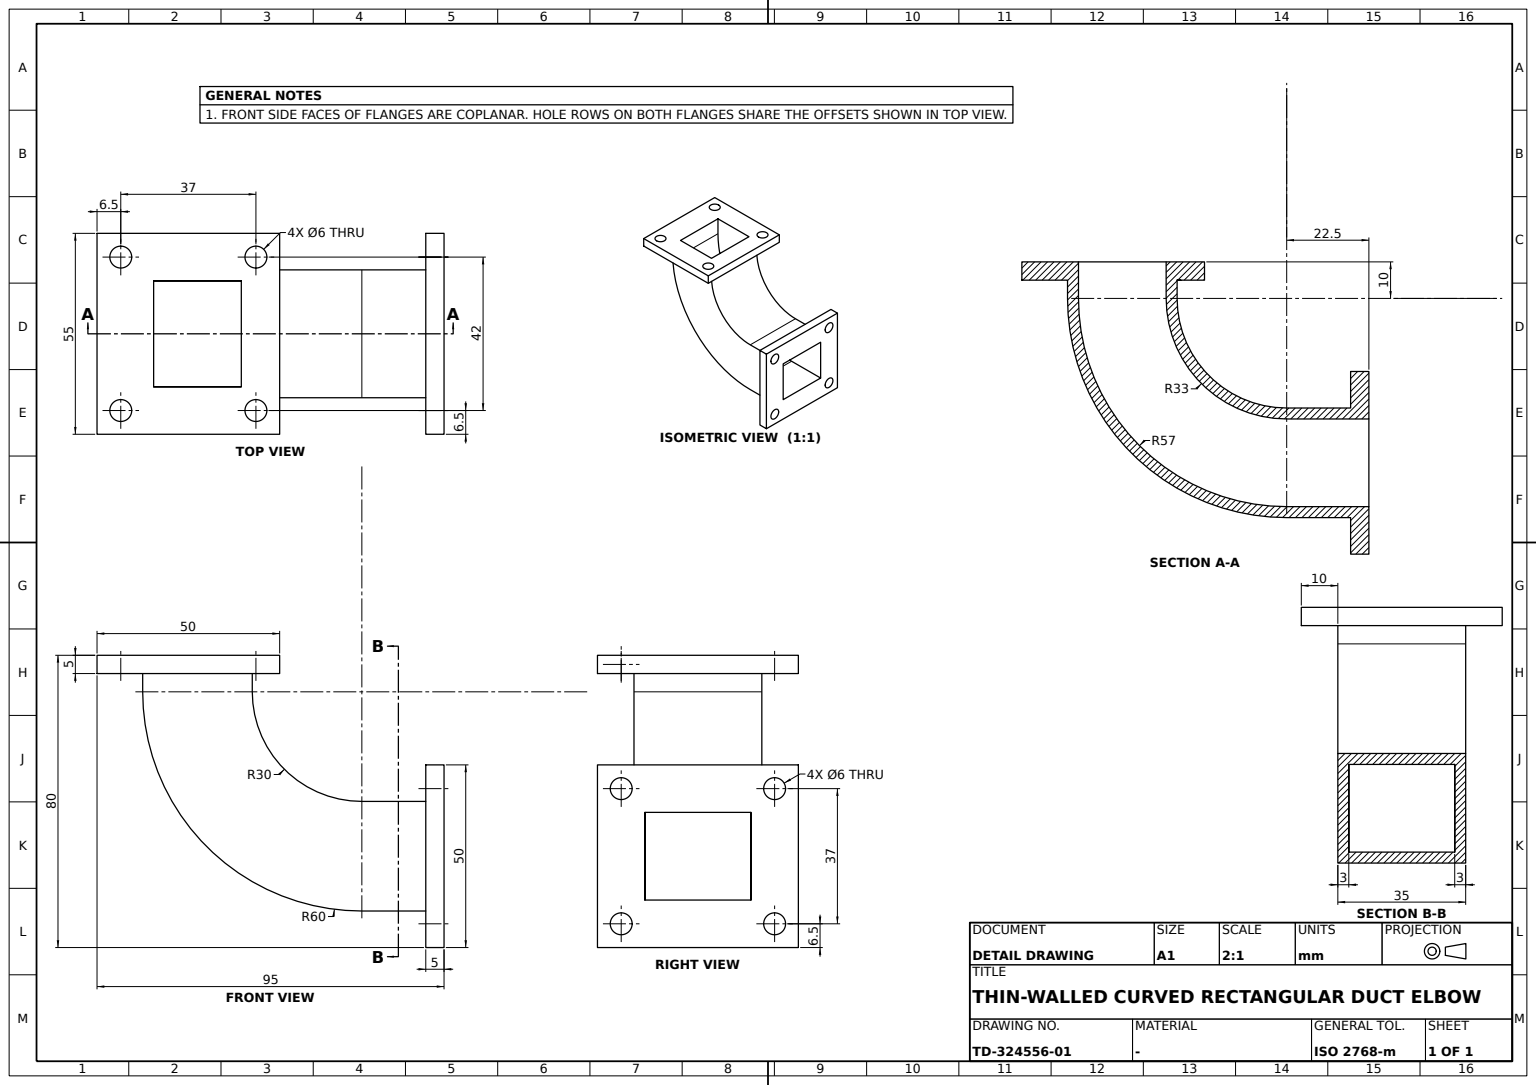
ISO-10303-21;
HEADER;
FILE_DESCRIPTION((''),'2;1');
FILE_NAME('','',(''),(''),'','','');
FILE_SCHEMA(('AUTOMOTIVE_DESIGN'));
ENDSEC;
DATA;
#1=APPLICATION_CONTEXT('');
#2=PRODUCT_CONTEXT('',#1,'mechanical');
#3=PRODUCT('','','',(#2));
#4=PRODUCT_DEFINITION_FORMATION('','',#3);
#5=PRODUCT_DEFINITION_CONTEXT('',#1,'design');
#6=PRODUCT_DEFINITION('','',#4,#5);
#7=PRODUCT_DEFINITION_SHAPE('','',#6);
#8=(LENGTH_UNIT()NAMED_UNIT(*)SI_UNIT(.MILLI.,.METRE.));
#9=(NAMED_UNIT(*)PLANE_ANGLE_UNIT()SI_UNIT($,.RADIAN.));
#10=(NAMED_UNIT(*)SI_UNIT($,.STERADIAN.)SOLID_ANGLE_UNIT());
#11=UNCERTAINTY_MEASURE_WITH_UNIT(LENGTH_MEASURE(1.E-05),#8,'distance_accuracy_value','');
#12=(GEOMETRIC_REPRESENTATION_CONTEXT(3)GLOBAL_UNCERTAINTY_ASSIGNED_CONTEXT((#11))GLOBAL_UNIT_ASSIGNED_CONTEXT((#8,#9,#10))REPRESENTATION_CONTEXT('',''));
#13=CARTESIAN_POINT('',(-24.,-18.5,0.));
#14=VERTEX_POINT('',#13);
#15=CARTESIAN_POINT('',(-18.,-18.5,0.));
#16=VERTEX_POINT('',#15);
#17=CARTESIAN_POINT('',(-21.,-18.5,0.));
#18=DIRECTION('',(0.,0.,-1.));
#19=DIRECTION('',(1.,0.,0.));
#20=AXIS2_PLACEMENT_3D('',#17,#18,#19);
#21=CIRCLE('',#20,3.);
#22=EDGE_CURVE('',#14,#16,#21,.T.);
#23=ORIENTED_EDGE('',*,*,#22,.F.);
#24=CARTESIAN_POINT('',(-24.,-18.5,-5.));
#25=VERTEX_POINT('',#24);
#26=CARTESIAN_POINT('',(-24.,-18.5,-2.5));
#27=DIRECTION('',(0.,0.,1.));
#28=VECTOR('',#27,1000.);
#29=LINE('',#26,#28);
#30=EDGE_CURVE('',#25,#14,#29,.T.);
#31=ORIENTED_EDGE('',*,*,#30,.F.);
#32=CARTESIAN_POINT('',(-18.,-18.5,-5.));
#33=VERTEX_POINT('',#32);
#34=CARTESIAN_POINT('',(-21.,-18.5,-5.));
#35=AXIS2_PLACEMENT_3D('',#34,#18,#19);
#36=CIRCLE('',#35,3.);
#37=EDGE_CURVE('',#25,#33,#36,.T.);
#38=ORIENTED_EDGE('',*,*,#37,.T.);
#39=CARTESIAN_POINT('',(-18.,-18.5,-2.5));
#40=LINE('',#39,#28);
#41=EDGE_CURVE('',#33,#16,#40,.T.);
#42=ORIENTED_EDGE('',*,*,#41,.T.);
#43=EDGE_LOOP('',(#23,#31,#38,#42));
#44=FACE_OUTER_BOUND('',#43,.T.);
#45=CARTESIAN_POINT('',(-21.,-18.5,-2.5));
#46=AXIS2_PLACEMENT_3D('',#45,#27,#19);
#47=CYLINDRICAL_SURFACE('',#46,3.);
#48=ADVANCED_FACE('',(#44),#47,.F.);
#49=CARTESIAN_POINT('',(-18.,-65.,31.5));
#50=VERTEX_POINT('',#49);
#51=CARTESIAN_POINT('',(-24.,-65.,31.5));
#52=VERTEX_POINT('',#51);
#53=CARTESIAN_POINT('',(-21.,-65.,31.5));
#54=DIRECTION('',(0.,-1.,0.));
#55=AXIS2_PLACEMENT_3D('',#53,#54,#19);
#56=CIRCLE('',#55,3.);
#57=EDGE_CURVE('',#50,#52,#56,.T.);
#58=ORIENTED_EDGE('',*,*,#57,.F.);
#59=CARTESIAN_POINT('',(-18.,-70.,31.5));
#60=VERTEX_POINT('',#59);
#61=CARTESIAN_POINT('',(-18.,-67.5,31.5));
#62=DIRECTION('',(0.,1.,0.));
#63=VECTOR('',#62,1000.);
#64=LINE('',#61,#63);
#65=EDGE_CURVE('',#60,#50,#64,.T.);
#66=ORIENTED_EDGE('',*,*,#65,.F.);
#67=CARTESIAN_POINT('',(-24.,-70.,31.5));
#68=VERTEX_POINT('',#67);
#69=CARTESIAN_POINT('',(-21.,-70.,31.5));
#70=AXIS2_PLACEMENT_3D('',#69,#54,#19);
#71=CIRCLE('',#70,3.);
#72=EDGE_CURVE('',#60,#68,#71,.T.);
#73=ORIENTED_EDGE('',*,*,#72,.T.);
#74=CARTESIAN_POINT('',(-24.,-67.5,31.5));
#75=LINE('',#74,#63);
#76=EDGE_CURVE('',#68,#52,#75,.T.);
#77=ORIENTED_EDGE('',*,*,#76,.T.);
#78=EDGE_LOOP('',(#58,#66,#73,#77));
#79=FACE_OUTER_BOUND('',#78,.T.);
#80=CARTESIAN_POINT('',(-21.,-67.5,31.5));
#81=AXIS2_PLACEMENT_3D('',#80,#62,#19);
#82=CYLINDRICAL_SURFACE('',#81,3.);
#83=ADVANCED_FACE('',(#79),#82,.F.);
#84=CARTESIAN_POINT('',(24.,-70.,68.5));
#85=VERTEX_POINT('',#84);
#86=CARTESIAN_POINT('',(24.,-65.,68.5));
#87=VERTEX_POINT('',#86);
#88=CARTESIAN_POINT('',(24.,-67.5,68.5));
#89=LINE('',#88,#63);
#90=EDGE_CURVE('',#85,#87,#89,.T.);
#91=ORIENTED_EDGE('',*,*,#90,.F.);
#92=CARTESIAN_POINT('',(18.,-70.,68.5));
#93=VERTEX_POINT('',#92);
#94=CARTESIAN_POINT('',(21.,-70.,68.5));
#95=AXIS2_PLACEMENT_3D('',#94,#54,#19);
#96=CIRCLE('',#95,3.);
#97=EDGE_CURVE('',#85,#93,#96,.T.);
#98=ORIENTED_EDGE('',*,*,#97,.T.);
#99=CARTESIAN_POINT('',(18.,-65.,68.5));
#100=VERTEX_POINT('',#99);
#101=CARTESIAN_POINT('',(18.,-67.5,68.5));
#102=LINE('',#101,#63);
#103=EDGE_CURVE('',#93,#100,#102,.T.);
#104=ORIENTED_EDGE('',*,*,#103,.T.);
#105=CARTESIAN_POINT('',(21.,-65.,68.5));
#106=AXIS2_PLACEMENT_3D('',#105,#54,#19);
#107=CIRCLE('',#106,3.);
#108=EDGE_CURVE('',#87,#100,#107,.T.);
#109=ORIENTED_EDGE('',*,*,#108,.F.);
#110=EDGE_LOOP('',(#91,#98,#104,#109));
#111=FACE_OUTER_BOUND('',#110,.T.);
#112=CARTESIAN_POINT('',(21.,-67.5,68.5));
#113=AXIS2_PLACEMENT_3D('',#112,#62,#19);
#114=CYLINDRICAL_SURFACE('',#113,3.);
#115=ADVANCED_FACE('',(#111),#114,.F.);
#116=ORIENTED_EDGE('',*,*,#108,.T.);
#117=EDGE_CURVE('',#100,#87,#107,.T.);
#118=ORIENTED_EDGE('',*,*,#117,.T.);
#119=EDGE_LOOP('',(#116,#118));
#120=FACE_BOUND('',#119,.T.);
#121=CARTESIAN_POINT('',(17.5,-65.,65.));
#122=VERTEX_POINT('',#121);
#123=CARTESIAN_POINT('',(-17.5,-65.,65.));
#124=VERTEX_POINT('',#123);
#125=CARTESIAN_POINT('',(0.,-65.,65.));
#126=DIRECTION('',(-1.,0.,0.));
#127=VECTOR('',#126,1000.);
#128=LINE('',#125,#127);
#129=EDGE_CURVE('',#122,#124,#128,.T.);
#130=ORIENTED_EDGE('',*,*,#129,.T.);
#131=CARTESIAN_POINT('',(-17.5,-65.,35.));
#132=VERTEX_POINT('',#131);
#133=CARTESIAN_POINT('',(-17.5,-65.,50.));
#134=VECTOR('',#18,1000.);
#135=LINE('',#133,#134);
#136=EDGE_CURVE('',#124,#132,#135,.T.);
#137=ORIENTED_EDGE('',*,*,#136,.T.);
#138=CARTESIAN_POINT('',(17.5,-65.,35.));
#139=VERTEX_POINT('',#138);
#140=CARTESIAN_POINT('',(0.,-65.,35.));
#141=VECTOR('',#19,1000.);
#142=LINE('',#140,#141);
#143=EDGE_CURVE('',#132,#139,#142,.T.);
#144=ORIENTED_EDGE('',*,*,#143,.T.);
#145=CARTESIAN_POINT('',(17.5,-65.,50.));
#146=LINE('',#145,#28);
#147=EDGE_CURVE('',#139,#122,#146,.T.);
#148=ORIENTED_EDGE('',*,*,#147,.T.);
#149=EDGE_LOOP('',(#130,#137,#144,#148));
#150=FACE_BOUND('',#149,.T.);
#151=CARTESIAN_POINT('',(-24.,-65.,68.5));
#152=VERTEX_POINT('',#151);
#153=CARTESIAN_POINT('',(-18.,-65.,68.5));
#154=VERTEX_POINT('',#153);
#155=CARTESIAN_POINT('',(-21.,-65.,68.5));
#156=AXIS2_PLACEMENT_3D('',#155,#54,#19);
#157=CIRCLE('',#156,3.);
#158=EDGE_CURVE('',#152,#154,#157,.T.);
#159=ORIENTED_EDGE('',*,*,#158,.T.);
#160=EDGE_CURVE('',#154,#152,#157,.T.);
#161=ORIENTED_EDGE('',*,*,#160,.T.);
#162=EDGE_LOOP('',(#159,#161));
#163=FACE_BOUND('',#162,.T.);
#164=CARTESIAN_POINT('',(-27.5,-65.,25.));
#165=VERTEX_POINT('',#164);
#166=CARTESIAN_POINT('',(27.5,-65.,25.));
#167=VERTEX_POINT('',#166);
#168=CARTESIAN_POINT('',(0.,-65.,25.));
#169=LINE('',#168,#141);
#170=EDGE_CURVE('',#165,#167,#169,.T.);
#171=ORIENTED_EDGE('',*,*,#170,.F.);
#172=CARTESIAN_POINT('',(-27.5,-65.,75.));
#173=VERTEX_POINT('',#172);
#174=CARTESIAN_POINT('',(-27.5,-65.,50.));
#175=LINE('',#174,#134);
#176=EDGE_CURVE('',#173,#165,#175,.T.);
#177=ORIENTED_EDGE('',*,*,#176,.F.);
#178=CARTESIAN_POINT('',(27.5,-65.,75.));
#179=VERTEX_POINT('',#178);
#180=CARTESIAN_POINT('',(0.,-65.,75.));
#181=LINE('',#180,#127);
#182=EDGE_CURVE('',#179,#173,#181,.T.);
#183=ORIENTED_EDGE('',*,*,#182,.F.);
#184=CARTESIAN_POINT('',(27.5,-65.,50.));
#185=LINE('',#184,#28);
#186=EDGE_CURVE('',#167,#179,#185,.T.);
#187=ORIENTED_EDGE('',*,*,#186,.F.);
#188=EDGE_LOOP('',(#171,#177,#183,#187));
#189=FACE_OUTER_BOUND('',#188,.T.);
#190=CARTESIAN_POINT('',(24.,-65.,31.5));
#191=VERTEX_POINT('',#190);
#192=CARTESIAN_POINT('',(18.,-65.,31.5));
#193=VERTEX_POINT('',#192);
#194=CARTESIAN_POINT('',(21.,-65.,31.5));
#195=AXIS2_PLACEMENT_3D('',#194,#54,#19);
#196=CIRCLE('',#195,3.);
#197=EDGE_CURVE('',#191,#193,#196,.T.);
#198=ORIENTED_EDGE('',*,*,#197,.T.);
#199=EDGE_CURVE('',#193,#191,#196,.T.);
#200=ORIENTED_EDGE('',*,*,#199,.T.);
#201=EDGE_LOOP('',(#198,#200));
#202=FACE_BOUND('',#201,.T.);
#203=EDGE_CURVE('',#52,#50,#56,.T.);
#204=ORIENTED_EDGE('',*,*,#203,.T.);
#205=ORIENTED_EDGE('',*,*,#57,.T.);
#206=EDGE_LOOP('',(#204,#205));
#207=FACE_BOUND('',#206,.T.);
#208=CARTESIAN_POINT('',(0.,-65.,0.));
#209=AXIS2_PLACEMENT_3D('',#208,#62,#126);
#210=PLANE('',#209);
#211=ADVANCED_FACE('',(#120,#150,#163,#189,#202,#207),#210,.T.);
#212=CARTESIAN_POINT('',(-27.5,25.,0.));
#213=VERTEX_POINT('',#212);
#214=CARTESIAN_POINT('',(-27.5,25.,-5.));
#215=VERTEX_POINT('',#214);
#216=CARTESIAN_POINT('',(-27.5,25.,-2.5));
#217=LINE('',#216,#134);
#218=EDGE_CURVE('',#213,#215,#217,.T.);
#219=ORIENTED_EDGE('',*,*,#218,.T.);
#220=CARTESIAN_POINT('',(-27.5,-25.,-5.));
#221=VERTEX_POINT('',#220);
#222=CARTESIAN_POINT('',(-27.5,0.,-5.));
#223=LINE('',#222,#63);
#224=EDGE_CURVE('',#221,#215,#223,.T.);
#225=ORIENTED_EDGE('',*,*,#224,.F.);
#226=CARTESIAN_POINT('',(-27.5,-25.,0.));
#227=VERTEX_POINT('',#226);
#228=CARTESIAN_POINT('',(-27.5,-25.,-2.5));
#229=LINE('',#228,#134);
#230=EDGE_CURVE('',#227,#221,#229,.T.);
#231=ORIENTED_EDGE('',*,*,#230,.F.);
#232=CARTESIAN_POINT('',(-27.5,0.,0.));
#233=LINE('',#232,#63);
#234=EDGE_CURVE('',#227,#213,#233,.T.);
#235=ORIENTED_EDGE('',*,*,#234,.T.);
#236=EDGE_LOOP('',(#219,#225,#231,#235));
#237=FACE_OUTER_BOUND('',#236,.T.);
#238=AXIS2_PLACEMENT_3D('',#164,#19,#27);
#239=PLANE('',#238);
#240=ADVANCED_FACE('',(#237),#239,.F.);
#241=CARTESIAN_POINT('',(-14.5,9.5,-5.));
#242=VERTEX_POINT('',#241);
#243=CARTESIAN_POINT('',(-14.5,9.5,5.));
#244=VERTEX_POINT('',#243);
#245=CARTESIAN_POINT('',(-14.5,9.5,0.));
#246=LINE('',#245,#28);
#247=EDGE_CURVE('',#242,#244,#246,.T.);
#248=ORIENTED_EDGE('',*,*,#247,.F.);
#249=CARTESIAN_POINT('',(14.5,9.5,-5.));
#250=VERTEX_POINT('',#249);
#251=CARTESIAN_POINT('',(0.,9.5,-5.));
#252=LINE('',#251,#141);
#253=EDGE_CURVE('',#242,#250,#252,.T.);
#254=ORIENTED_EDGE('',*,*,#253,.T.);
#255=CARTESIAN_POINT('',(14.5,9.5,5.));
#256=VERTEX_POINT('',#255);
#257=CARTESIAN_POINT('',(14.5,9.5,0.));
#258=LINE('',#257,#28);
#259=EDGE_CURVE('',#250,#256,#258,.T.);
#260=ORIENTED_EDGE('',*,*,#259,.T.);
#261=CARTESIAN_POINT('',(0.,9.5,5.));
#262=LINE('',#261,#127);
#263=EDGE_CURVE('',#256,#244,#262,.T.);
#264=ORIENTED_EDGE('',*,*,#263,.T.);
#265=EDGE_LOOP('',(#248,#254,#260,#264));
#266=FACE_OUTER_BOUND('',#265,.T.);
#267=AXIS2_PLACEMENT_3D('',#257,#62,#126);
#268=PLANE('',#267);
#269=ADVANCED_FACE('',(#266),#268,.F.);
#270=CARTESIAN_POINT('',(-14.5,-14.5,-5.));
#271=VERTEX_POINT('',#270);
#272=CARTESIAN_POINT('',(-14.5,-14.5,5.));
#273=VERTEX_POINT('',#272);
#274=CARTESIAN_POINT('',(-14.5,-14.5,0.));
#275=LINE('',#274,#28);
#276=EDGE_CURVE('',#271,#273,#275,.T.);
#277=ORIENTED_EDGE('',*,*,#276,.T.);
#278=CARTESIAN_POINT('',(14.5,-14.5,5.));
#279=VERTEX_POINT('',#278);
#280=CARTESIAN_POINT('',(0.,-14.5,5.));
#281=LINE('',#280,#141);
#282=EDGE_CURVE('',#273,#279,#281,.T.);
#283=ORIENTED_EDGE('',*,*,#282,.T.);
#284=CARTESIAN_POINT('',(14.5,-14.5,-5.));
#285=VERTEX_POINT('',#284);
#286=CARTESIAN_POINT('',(14.5,-14.5,0.));
#287=LINE('',#286,#28);
#288=EDGE_CURVE('',#285,#279,#287,.T.);
#289=ORIENTED_EDGE('',*,*,#288,.F.);
#290=CARTESIAN_POINT('',(0.,-14.5,-5.));
#291=LINE('',#290,#127);
#292=EDGE_CURVE('',#285,#271,#291,.T.);
#293=ORIENTED_EDGE('',*,*,#292,.T.);
#294=EDGE_LOOP('',(#277,#283,#289,#293));
#295=FACE_OUTER_BOUND('',#294,.T.);
#296=AXIS2_PLACEMENT_3D('',#274,#54,#19);
#297=PLANE('',#296);
#298=ADVANCED_FACE('',(#295),#297,.F.);
#299=CARTESIAN_POINT('',(-18.,-70.,68.5));
#300=VERTEX_POINT('',#299);
#301=CARTESIAN_POINT('',(-18.,-67.5,68.5));
#302=LINE('',#301,#63);
#303=EDGE_CURVE('',#300,#154,#302,.T.);
#304=ORIENTED_EDGE('',*,*,#303,.F.);
#305=CARTESIAN_POINT('',(-24.,-70.,68.5));
#306=VERTEX_POINT('',#305);
#307=CARTESIAN_POINT('',(-21.,-70.,68.5));
#308=AXIS2_PLACEMENT_3D('',#307,#54,#19);
#309=CIRCLE('',#308,3.);
#310=EDGE_CURVE('',#300,#306,#309,.T.);
#311=ORIENTED_EDGE('',*,*,#310,.T.);
#312=CARTESIAN_POINT('',(-24.,-67.5,68.5));
#313=LINE('',#312,#63);
#314=EDGE_CURVE('',#306,#152,#313,.T.);
#315=ORIENTED_EDGE('',*,*,#314,.T.);
#316=ORIENTED_EDGE('',*,*,#160,.F.);
#317=EDGE_LOOP('',(#304,#311,#315,#316));
#318=FACE_OUTER_BOUND('',#317,.T.);
#319=CARTESIAN_POINT('',(-21.,-67.5,68.5));
#320=AXIS2_PLACEMENT_3D('',#319,#62,#19);
#321=CYLINDRICAL_SURFACE('',#320,3.);
#322=ADVANCED_FACE('',(#318),#321,.F.);
#323=CARTESIAN_POINT('',(-14.5,-70.,38.));
#324=VERTEX_POINT('',#323);
#325=CARTESIAN_POINT('',(-14.5,-47.5,38.));
#326=VERTEX_POINT('',#325);
#327=CARTESIAN_POINT('',(-14.5,-58.75,38.));
#328=LINE('',#327,#63);
#329=EDGE_CURVE('',#324,#326,#328,.T.);
#330=ORIENTED_EDGE('',*,*,#329,.F.);
#331=CARTESIAN_POINT('',(14.5,-70.,38.));
#332=VERTEX_POINT('',#331);
#333=CARTESIAN_POINT('',(0.,-70.,38.));
#334=LINE('',#333,#141);
#335=EDGE_CURVE('',#324,#332,#334,.T.);
#336=ORIENTED_EDGE('',*,*,#335,.T.);
#337=CARTESIAN_POINT('',(14.5,-47.5,38.));
#338=VERTEX_POINT('',#337);
#339=CARTESIAN_POINT('',(14.5,-58.75,38.));
#340=LINE('',#339,#63);
#341=EDGE_CURVE('',#332,#338,#340,.T.);
#342=ORIENTED_EDGE('',*,*,#341,.T.);
#343=CARTESIAN_POINT('',(0.,-47.5,38.));
#344=LINE('',#343,#141);
#345=EDGE_CURVE('',#326,#338,#344,.T.);
#346=ORIENTED_EDGE('',*,*,#345,.F.);
#347=EDGE_LOOP('',(#330,#336,#342,#346));
#348=FACE_OUTER_BOUND('',#347,.T.);
#349=CARTESIAN_POINT('',(-14.5,-65.,38.));
#350=AXIS2_PLACEMENT_3D('',#349,#27,#19);
#351=PLANE('',#350);
#352=ADVANCED_FACE('',(#348),#351,.T.);
#353=ORIENTED_EDGE('',*,*,#263,.F.);
#354=CARTESIAN_POINT('',(14.5,-47.5,62.));
#355=VERTEX_POINT('',#354);
#356=CARTESIAN_POINT('',(14.5,-47.5,5.));
#357=AXIS2_PLACEMENT_3D('',#356,#19,#62);
#358=CIRCLE('',#357,57.);
#359=EDGE_CURVE('',#256,#355,#358,.T.);
#360=ORIENTED_EDGE('',*,*,#359,.T.);
#361=CARTESIAN_POINT('',(-14.5,-47.5,62.));
#362=VERTEX_POINT('',#361);
#363=CARTESIAN_POINT('',(0.,-47.5,62.));
#364=LINE('',#363,#127);
#365=EDGE_CURVE('',#355,#362,#364,.T.);
#366=ORIENTED_EDGE('',*,*,#365,.T.);
#367=CARTESIAN_POINT('',(-14.5,-47.5,5.));
#368=AXIS2_PLACEMENT_3D('',#367,#19,#62);
#369=CIRCLE('',#368,57.);
#370=EDGE_CURVE('',#244,#362,#369,.T.);
#371=ORIENTED_EDGE('',*,*,#370,.F.);
#372=EDGE_LOOP('',(#353,#360,#366,#371));
#373=FACE_OUTER_BOUND('',#372,.T.);
#374=CARTESIAN_POINT('',(0.,-47.5,5.));
#375=AXIS2_PLACEMENT_3D('',#374,#126,#62);
#376=CYLINDRICAL_SURFACE('',#375,57.);
#377=ADVANCED_FACE('',(#373),#376,.F.);
#378=CARTESIAN_POINT('',(-24.,18.5,-5.));
#379=VERTEX_POINT('',#378);
#380=CARTESIAN_POINT('',(-24.,18.5,0.));
#381=VERTEX_POINT('',#380);
#382=CARTESIAN_POINT('',(-24.,18.5,-2.5));
#383=LINE('',#382,#28);
#384=EDGE_CURVE('',#379,#381,#383,.T.);
#385=ORIENTED_EDGE('',*,*,#384,.F.);
#386=CARTESIAN_POINT('',(-18.,18.5,-5.));
#387=VERTEX_POINT('',#386);
#388=CARTESIAN_POINT('',(-21.,18.5,-5.));
#389=AXIS2_PLACEMENT_3D('',#388,#18,#19);
#390=CIRCLE('',#389,3.);
#391=EDGE_CURVE('',#379,#387,#390,.T.);
#392=ORIENTED_EDGE('',*,*,#391,.T.);
#393=CARTESIAN_POINT('',(-18.,18.5,0.));
#394=VERTEX_POINT('',#393);
#395=CARTESIAN_POINT('',(-18.,18.5,-2.5));
#396=LINE('',#395,#28);
#397=EDGE_CURVE('',#387,#394,#396,.T.);
#398=ORIENTED_EDGE('',*,*,#397,.T.);
#399=CARTESIAN_POINT('',(-21.,18.5,0.));
#400=AXIS2_PLACEMENT_3D('',#399,#18,#19);
#401=CIRCLE('',#400,3.);
#402=EDGE_CURVE('',#381,#394,#401,.T.);
#403=ORIENTED_EDGE('',*,*,#402,.F.);
#404=EDGE_LOOP('',(#385,#392,#398,#403));
#405=FACE_OUTER_BOUND('',#404,.T.);
#406=CARTESIAN_POINT('',(-21.,18.5,-2.5));
#407=AXIS2_PLACEMENT_3D('',#406,#27,#19);
#408=CYLINDRICAL_SURFACE('',#407,3.);
#409=ADVANCED_FACE('',(#405),#408,.F.);
#410=CARTESIAN_POINT('',(24.,-70.,31.5));
#411=VERTEX_POINT('',#410);
#412=CARTESIAN_POINT('',(18.,-70.,31.5));
#413=VERTEX_POINT('',#412);
#414=CARTESIAN_POINT('',(21.,-70.,31.5));
#415=AXIS2_PLACEMENT_3D('',#414,#54,#19);
#416=CIRCLE('',#415,3.);
#417=EDGE_CURVE('',#411,#413,#416,.T.);
#418=ORIENTED_EDGE('',*,*,#417,.T.);
#419=CARTESIAN_POINT('',(18.,-67.5,31.5));
#420=LINE('',#419,#63);
#421=EDGE_CURVE('',#413,#193,#420,.T.);
#422=ORIENTED_EDGE('',*,*,#421,.T.);
#423=ORIENTED_EDGE('',*,*,#197,.F.);
#424=CARTESIAN_POINT('',(24.,-67.5,31.5));
#425=LINE('',#424,#63);
#426=EDGE_CURVE('',#411,#191,#425,.T.);
#427=ORIENTED_EDGE('',*,*,#426,.F.);
#428=EDGE_LOOP('',(#418,#422,#423,#427));
#429=FACE_OUTER_BOUND('',#428,.T.);
#430=CARTESIAN_POINT('',(21.,-67.5,31.5));
#431=AXIS2_PLACEMENT_3D('',#430,#62,#19);
#432=CYLINDRICAL_SURFACE('',#431,3.);
#433=ADVANCED_FACE('',(#429),#432,.F.);
#434=CARTESIAN_POINT('',(14.5,-70.,62.));
#435=VERTEX_POINT('',#434);
#436=CARTESIAN_POINT('',(-14.5,-70.,62.));
#437=VERTEX_POINT('',#436);
#438=CARTESIAN_POINT('',(0.,-70.,62.));
#439=LINE('',#438,#127);
#440=EDGE_CURVE('',#435,#437,#439,.T.);
#441=ORIENTED_EDGE('',*,*,#440,.T.);
#442=CARTESIAN_POINT('',(-14.5,-58.75,62.));
#443=LINE('',#442,#63);
#444=EDGE_CURVE('',#437,#362,#443,.T.);
#445=ORIENTED_EDGE('',*,*,#444,.T.);
#446=ORIENTED_EDGE('',*,*,#365,.F.);
#447=CARTESIAN_POINT('',(14.5,-58.75,62.));
#448=LINE('',#447,#63);
#449=EDGE_CURVE('',#435,#355,#448,.T.);
#450=ORIENTED_EDGE('',*,*,#449,.F.);
#451=EDGE_LOOP('',(#441,#445,#446,#450));
#452=FACE_OUTER_BOUND('',#451,.T.);
#453=CARTESIAN_POINT('',(14.5,-65.,62.));
#454=AXIS2_PLACEMENT_3D('',#453,#18,#126);
#455=PLANE('',#454);
#456=ADVANCED_FACE('',(#452),#455,.T.);
#457=CARTESIAN_POINT('',(-17.5,-17.5,5.));
#458=VERTEX_POINT('',#457);
#459=CARTESIAN_POINT('',(-17.5,-47.5,35.));
#460=VERTEX_POINT('',#459);
#461=CARTESIAN_POINT('',(-17.5,-47.5,5.));
#462=AXIS2_PLACEMENT_3D('',#461,#19,#62);
#463=CIRCLE('',#462,30.);
#464=EDGE_CURVE('',#458,#460,#463,.T.);
#465=ORIENTED_EDGE('',*,*,#464,.T.);
#466=CARTESIAN_POINT('',(-17.5,-56.25,35.));
#467=LINE('',#466,#63);
#468=EDGE_CURVE('',#132,#460,#467,.T.);
#469=ORIENTED_EDGE('',*,*,#468,.F.);
#470=ORIENTED_EDGE('',*,*,#136,.F.);
#471=CARTESIAN_POINT('',(-17.5,-47.5,65.));
#472=VERTEX_POINT('',#471);
#473=CARTESIAN_POINT('',(-17.5,-56.25,65.));
#474=LINE('',#473,#63);
#475=EDGE_CURVE('',#124,#472,#474,.T.);
#476=ORIENTED_EDGE('',*,*,#475,.T.);
#477=CARTESIAN_POINT('',(-17.5,12.5,5.));
#478=VERTEX_POINT('',#477);
#479=CIRCLE('',#462,60.);
#480=EDGE_CURVE('',#478,#472,#479,.T.);
#481=ORIENTED_EDGE('',*,*,#480,.F.);
#482=CARTESIAN_POINT('',(-17.5,12.5,0.));
#483=VERTEX_POINT('',#482);
#484=CARTESIAN_POINT('',(-17.5,12.5,2.5));
#485=LINE('',#484,#28);
#486=EDGE_CURVE('',#483,#478,#485,.T.);
#487=ORIENTED_EDGE('',*,*,#486,.F.);
#488=CARTESIAN_POINT('',(-17.5,-17.5,0.));
#489=VERTEX_POINT('',#488);
#490=CARTESIAN_POINT('',(-17.5,-2.5,0.));
#491=VECTOR('',#54,1000.);
#492=LINE('',#490,#491);
#493=EDGE_CURVE('',#483,#489,#492,.T.);
#494=ORIENTED_EDGE('',*,*,#493,.T.);
#495=CARTESIAN_POINT('',(-17.5,-17.5,2.5));
#496=LINE('',#495,#28);
#497=EDGE_CURVE('',#489,#458,#496,.T.);
#498=ORIENTED_EDGE('',*,*,#497,.T.);
#499=EDGE_LOOP('',(#465,#469,#470,#476,#481,#487,#494,#498));
#500=FACE_OUTER_BOUND('',#499,.T.);
#501=AXIS2_PLACEMENT_3D('',#482,#126,#54);
#502=PLANE('',#501);
#503=ADVANCED_FACE('',(#500),#502,.T.);
#504=ORIENTED_EDGE('',*,*,#303,.T.);
#505=ORIENTED_EDGE('',*,*,#158,.F.);
#506=ORIENTED_EDGE('',*,*,#314,.F.);
#507=EDGE_CURVE('',#306,#300,#309,.T.);
#508=ORIENTED_EDGE('',*,*,#507,.T.);
#509=EDGE_LOOP('',(#504,#505,#506,#508));
#510=FACE_OUTER_BOUND('',#509,.T.);
#511=ADVANCED_FACE('',(#510),#321,.F.);
#512=CARTESIAN_POINT('',(27.5,25.,0.));
#513=VERTEX_POINT('',#512);
#514=CARTESIAN_POINT('',(27.5,-25.,0.));
#515=VERTEX_POINT('',#514);
#516=CARTESIAN_POINT('',(27.5,0.,0.));
#517=LINE('',#516,#491);
#518=EDGE_CURVE('',#513,#515,#517,.T.);
#519=ORIENTED_EDGE('',*,*,#518,.T.);
#520=CARTESIAN_POINT('',(27.5,-25.,-5.));
#521=VERTEX_POINT('',#520);
#522=CARTESIAN_POINT('',(27.5,-25.,-2.5));
#523=LINE('',#522,#134);
#524=EDGE_CURVE('',#515,#521,#523,.T.);
#525=ORIENTED_EDGE('',*,*,#524,.T.);
#526=CARTESIAN_POINT('',(27.5,25.,-5.));
#527=VERTEX_POINT('',#526);
#528=CARTESIAN_POINT('',(27.5,0.,-5.));
#529=LINE('',#528,#491);
#530=EDGE_CURVE('',#527,#521,#529,.T.);
#531=ORIENTED_EDGE('',*,*,#530,.F.);
#532=CARTESIAN_POINT('',(27.5,25.,-2.5));
#533=LINE('',#532,#134);
#534=EDGE_CURVE('',#513,#527,#533,.T.);
#535=ORIENTED_EDGE('',*,*,#534,.F.);
#536=EDGE_LOOP('',(#519,#525,#531,#535));
#537=FACE_OUTER_BOUND('',#536,.T.);
#538=AXIS2_PLACEMENT_3D('',#178,#126,#18);
#539=PLANE('',#538);
#540=ADVANCED_FACE('',(#537),#539,.F.);
#541=CARTESIAN_POINT('',(24.,-18.5,0.));
#542=VERTEX_POINT('',#541);
#543=CARTESIAN_POINT('',(18.,-18.5,0.));
#544=VERTEX_POINT('',#543);
#545=CARTESIAN_POINT('',(21.,-18.5,0.));
#546=AXIS2_PLACEMENT_3D('',#545,#18,#19);
#547=CIRCLE('',#546,3.);
#548=EDGE_CURVE('',#542,#544,#547,.T.);
#549=ORIENTED_EDGE('',*,*,#548,.T.);
#550=EDGE_CURVE('',#544,#542,#547,.T.);
#551=ORIENTED_EDGE('',*,*,#550,.T.);
#552=EDGE_LOOP('',(#549,#551));
#553=FACE_BOUND('',#552,.T.);
#554=EDGE_CURVE('',#394,#381,#401,.T.);
#555=ORIENTED_EDGE('',*,*,#554,.T.);
#556=ORIENTED_EDGE('',*,*,#402,.T.);
#557=EDGE_LOOP('',(#555,#556));
#558=FACE_BOUND('',#557,.T.);
#559=EDGE_CURVE('',#16,#14,#21,.T.);
#560=ORIENTED_EDGE('',*,*,#559,.T.);
#561=ORIENTED_EDGE('',*,*,#22,.T.);
#562=EDGE_LOOP('',(#560,#561));
#563=FACE_BOUND('',#562,.T.);
#564=CARTESIAN_POINT('',(17.5,12.5,0.));
#565=VERTEX_POINT('',#564);
#566=CARTESIAN_POINT('',(0.,12.5,0.));
#567=LINE('',#566,#127);
#568=EDGE_CURVE('',#565,#483,#567,.T.);
#569=ORIENTED_EDGE('',*,*,#568,.F.);
#570=CARTESIAN_POINT('',(17.5,-17.5,0.));
#571=VERTEX_POINT('',#570);
#572=CARTESIAN_POINT('',(17.5,-2.5,0.));
#573=LINE('',#572,#63);
#574=EDGE_CURVE('',#571,#565,#573,.T.);
#575=ORIENTED_EDGE('',*,*,#574,.F.);
#576=CARTESIAN_POINT('',(0.,-17.5,0.));
#577=LINE('',#576,#141);
#578=EDGE_CURVE('',#489,#571,#577,.T.);
#579=ORIENTED_EDGE('',*,*,#578,.F.);
#580=ORIENTED_EDGE('',*,*,#493,.F.);
#581=EDGE_LOOP('',(#569,#575,#579,#580));
#582=FACE_BOUND('',#581,.T.);
#583=CARTESIAN_POINT('',(0.,25.,0.));
#584=LINE('',#583,#141);
#585=EDGE_CURVE('',#213,#513,#584,.T.);
#586=ORIENTED_EDGE('',*,*,#585,.F.);
#587=ORIENTED_EDGE('',*,*,#234,.F.);
#588=CARTESIAN_POINT('',(0.,-25.,0.));
#589=LINE('',#588,#127);
#590=EDGE_CURVE('',#515,#227,#589,.T.);
#591=ORIENTED_EDGE('',*,*,#590,.F.);
#592=ORIENTED_EDGE('',*,*,#518,.F.);
#593=EDGE_LOOP('',(#586,#587,#591,#592));
#594=FACE_OUTER_BOUND('',#593,.T.);
#595=CARTESIAN_POINT('',(18.,18.5,0.));
#596=VERTEX_POINT('',#595);
#597=CARTESIAN_POINT('',(24.,18.5,0.));
#598=VERTEX_POINT('',#597);
#599=CARTESIAN_POINT('',(21.,18.5,0.));
#600=AXIS2_PLACEMENT_3D('',#599,#18,#19);
#601=CIRCLE('',#600,3.);
#602=EDGE_CURVE('',#596,#598,#601,.T.);
#603=ORIENTED_EDGE('',*,*,#602,.T.);
#604=EDGE_CURVE('',#598,#596,#601,.T.);
#605=ORIENTED_EDGE('',*,*,#604,.T.);
#606=EDGE_LOOP('',(#603,#605));
#607=FACE_BOUND('',#606,.T.);
#608=CARTESIAN_POINT('',(0.,-52.5,0.));
#609=AXIS2_PLACEMENT_3D('',#608,#18,#126);
#610=PLANE('',#609);
#611=ADVANCED_FACE('',(#553,#558,#563,#582,#594,#607),#610,.F.);
#612=ORIENTED_EDGE('',*,*,#449,.T.);
#613=ORIENTED_EDGE('',*,*,#359,.F.);
#614=ORIENTED_EDGE('',*,*,#259,.F.);
#615=CARTESIAN_POINT('',(14.5,-2.5,-5.));
#616=LINE('',#615,#491);
#617=EDGE_CURVE('',#250,#285,#616,.T.);
#618=ORIENTED_EDGE('',*,*,#617,.T.);
#619=ORIENTED_EDGE('',*,*,#288,.T.);
#620=CIRCLE('',#357,33.);
#621=EDGE_CURVE('',#279,#338,#620,.T.);
#622=ORIENTED_EDGE('',*,*,#621,.T.);
#623=ORIENTED_EDGE('',*,*,#341,.F.);
#624=CARTESIAN_POINT('',(14.5,-70.,50.));
#625=LINE('',#624,#28);
#626=EDGE_CURVE('',#332,#435,#625,.T.);
#627=ORIENTED_EDGE('',*,*,#626,.T.);
#628=EDGE_LOOP('',(#612,#613,#614,#618,#619,#622,#623,#627));
#629=FACE_OUTER_BOUND('',#628,.T.);
#630=AXIS2_PLACEMENT_3D('',#286,#19,#62);
#631=PLANE('',#630);
#632=ADVANCED_FACE('',(#629),#631,.F.);
#633=ORIENTED_EDGE('',*,*,#534,.T.);
#634=CARTESIAN_POINT('',(0.,25.,-5.));
#635=LINE('',#634,#141);
#636=EDGE_CURVE('',#215,#527,#635,.T.);
#637=ORIENTED_EDGE('',*,*,#636,.F.);
#638=ORIENTED_EDGE('',*,*,#218,.F.);
#639=ORIENTED_EDGE('',*,*,#585,.T.);
#640=EDGE_LOOP('',(#633,#637,#638,#639));
#641=FACE_OUTER_BOUND('',#640,.T.);
#642=AXIS2_PLACEMENT_3D('',#512,#54,#126);
#643=PLANE('',#642);
#644=ADVANCED_FACE('',(#641),#643,.F.);
#645=CARTESIAN_POINT('',(24.,-18.5,-5.));
#646=VERTEX_POINT('',#645);
#647=CARTESIAN_POINT('',(24.,-18.5,-2.5));
#648=LINE('',#647,#28);
#649=EDGE_CURVE('',#646,#542,#648,.T.);
#650=ORIENTED_EDGE('',*,*,#649,.T.);
#651=ORIENTED_EDGE('',*,*,#550,.F.);
#652=CARTESIAN_POINT('',(18.,-18.5,-5.));
#653=VERTEX_POINT('',#652);
#654=CARTESIAN_POINT('',(18.,-18.5,-2.5));
#655=LINE('',#654,#28);
#656=EDGE_CURVE('',#653,#544,#655,.T.);
#657=ORIENTED_EDGE('',*,*,#656,.F.);
#658=CARTESIAN_POINT('',(21.,-18.5,-5.));
#659=AXIS2_PLACEMENT_3D('',#658,#18,#19);
#660=CIRCLE('',#659,3.);
#661=EDGE_CURVE('',#653,#646,#660,.T.);
#662=ORIENTED_EDGE('',*,*,#661,.T.);
#663=EDGE_LOOP('',(#650,#651,#657,#662));
#664=FACE_OUTER_BOUND('',#663,.T.);
#665=CARTESIAN_POINT('',(21.,-18.5,-2.5));
#666=AXIS2_PLACEMENT_3D('',#665,#27,#19);
#667=CYLINDRICAL_SURFACE('',#666,3.);
#668=ADVANCED_FACE('',(#664),#667,.F.);
#669=ORIENTED_EDGE('',*,*,#444,.F.);
#670=CARTESIAN_POINT('',(-14.5,-70.,50.));
#671=LINE('',#670,#134);
#672=EDGE_CURVE('',#437,#324,#671,.T.);
#673=ORIENTED_EDGE('',*,*,#672,.T.);
#674=ORIENTED_EDGE('',*,*,#329,.T.);
#675=CIRCLE('',#368,33.);
#676=EDGE_CURVE('',#273,#326,#675,.T.);
#677=ORIENTED_EDGE('',*,*,#676,.F.);
#678=ORIENTED_EDGE('',*,*,#276,.F.);
#679=CARTESIAN_POINT('',(-14.5,-2.5,-5.));
#680=LINE('',#679,#63);
#681=EDGE_CURVE('',#271,#242,#680,.T.);
#682=ORIENTED_EDGE('',*,*,#681,.T.);
#683=ORIENTED_EDGE('',*,*,#247,.T.);
#684=ORIENTED_EDGE('',*,*,#370,.T.);
#685=EDGE_LOOP('',(#669,#673,#674,#677,#678,#682,#683,#684));
#686=FACE_OUTER_BOUND('',#685,.T.);
#687=AXIS2_PLACEMENT_3D('',#245,#126,#54);
#688=PLANE('',#687);
#689=ADVANCED_FACE('',(#686),#688,.F.);
#690=ORIENTED_EDGE('',*,*,#203,.F.);
#691=ORIENTED_EDGE('',*,*,#76,.F.);
#692=EDGE_CURVE('',#68,#60,#71,.T.);
#693=ORIENTED_EDGE('',*,*,#692,.T.);
#694=ORIENTED_EDGE('',*,*,#65,.T.);
#695=EDGE_LOOP('',(#690,#691,#693,#694));
#696=FACE_OUTER_BOUND('',#695,.T.);
#697=ADVANCED_FACE('',(#696),#82,.F.);
#698=ORIENTED_EDGE('',*,*,#554,.F.);
#699=ORIENTED_EDGE('',*,*,#397,.F.);
#700=EDGE_CURVE('',#387,#379,#390,.T.);
#701=ORIENTED_EDGE('',*,*,#700,.T.);
#702=ORIENTED_EDGE('',*,*,#384,.T.);
#703=EDGE_LOOP('',(#698,#699,#701,#702));
#704=FACE_OUTER_BOUND('',#703,.T.);
#705=ADVANCED_FACE('',(#704),#408,.F.);
#706=ORIENTED_EDGE('',*,*,#661,.F.);
#707=EDGE_CURVE('',#646,#653,#660,.T.);
#708=ORIENTED_EDGE('',*,*,#707,.F.);
#709=EDGE_LOOP('',(#706,#708));
#710=FACE_BOUND('',#709,.T.);
#711=ORIENTED_EDGE('',*,*,#700,.F.);
#712=ORIENTED_EDGE('',*,*,#391,.F.);
#713=EDGE_LOOP('',(#711,#712));
#714=FACE_BOUND('',#713,.T.);
#715=ORIENTED_EDGE('',*,*,#292,.F.);
#716=ORIENTED_EDGE('',*,*,#617,.F.);
#717=ORIENTED_EDGE('',*,*,#253,.F.);
#718=ORIENTED_EDGE('',*,*,#681,.F.);
#719=EDGE_LOOP('',(#715,#716,#717,#718));
#720=FACE_BOUND('',#719,.T.);
#721=ORIENTED_EDGE('',*,*,#530,.T.);
#722=CARTESIAN_POINT('',(0.,-25.,-5.));
#723=LINE('',#722,#127);
#724=EDGE_CURVE('',#521,#221,#723,.T.);
#725=ORIENTED_EDGE('',*,*,#724,.T.);
#726=ORIENTED_EDGE('',*,*,#224,.T.);
#727=ORIENTED_EDGE('',*,*,#636,.T.);
#728=EDGE_LOOP('',(#721,#725,#726,#727));
#729=FACE_OUTER_BOUND('',#728,.T.);
#730=CARTESIAN_POINT('',(24.,18.5,-5.));
#731=VERTEX_POINT('',#730);
#732=CARTESIAN_POINT('',(18.,18.5,-5.));
#733=VERTEX_POINT('',#732);
#734=CARTESIAN_POINT('',(21.,18.5,-5.));
#735=AXIS2_PLACEMENT_3D('',#734,#18,#19);
#736=CIRCLE('',#735,3.);
#737=EDGE_CURVE('',#731,#733,#736,.T.);
#738=ORIENTED_EDGE('',*,*,#737,.F.);
#739=EDGE_CURVE('',#733,#731,#736,.T.);
#740=ORIENTED_EDGE('',*,*,#739,.F.);
#741=EDGE_LOOP('',(#738,#740));
#742=FACE_BOUND('',#741,.T.);
#743=EDGE_CURVE('',#33,#25,#36,.T.);
#744=ORIENTED_EDGE('',*,*,#743,.F.);
#745=ORIENTED_EDGE('',*,*,#37,.F.);
#746=EDGE_LOOP('',(#744,#745));
#747=FACE_BOUND('',#746,.T.);
#748=CARTESIAN_POINT('',(0.,0.,-5.));
#749=AXIS2_PLACEMENT_3D('',#748,#18,#19);
#750=PLANE('',#749);
#751=ADVANCED_FACE('',(#710,#714,#720,#729,#742,#747),#750,.T.);
#752=CARTESIAN_POINT('',(27.5,-70.,25.));
#753=VERTEX_POINT('',#752);
#754=CARTESIAN_POINT('',(27.5,-70.,75.));
#755=VERTEX_POINT('',#754);
#756=CARTESIAN_POINT('',(27.5,-70.,50.));
#757=LINE('',#756,#28);
#758=EDGE_CURVE('',#753,#755,#757,.T.);
#759=ORIENTED_EDGE('',*,*,#758,.F.);
#760=CARTESIAN_POINT('',(27.5,-67.5,25.));
#761=LINE('',#760,#491);
#762=EDGE_CURVE('',#167,#753,#761,.T.);
#763=ORIENTED_EDGE('',*,*,#762,.F.);
#764=ORIENTED_EDGE('',*,*,#186,.T.);
#765=CARTESIAN_POINT('',(27.5,-67.5,75.));
#766=LINE('',#765,#491);
#767=EDGE_CURVE('',#179,#755,#766,.T.);
#768=ORIENTED_EDGE('',*,*,#767,.T.);
#769=EDGE_LOOP('',(#759,#763,#764,#768));
#770=FACE_OUTER_BOUND('',#769,.T.);
#771=ADVANCED_FACE('',(#770),#539,.F.);
#772=CARTESIAN_POINT('',(17.5,-47.5,35.));
#773=VERTEX_POINT('',#772);
#774=CARTESIAN_POINT('',(17.5,-56.25,35.));
#775=LINE('',#774,#63);
#776=EDGE_CURVE('',#139,#773,#775,.T.);
#777=ORIENTED_EDGE('',*,*,#776,.F.);
#778=ORIENTED_EDGE('',*,*,#143,.F.);
#779=ORIENTED_EDGE('',*,*,#468,.T.);
#780=CARTESIAN_POINT('',(0.,-47.5,35.));
#781=LINE('',#780,#141);
#782=EDGE_CURVE('',#460,#773,#781,.T.);
#783=ORIENTED_EDGE('',*,*,#782,.T.);
#784=EDGE_LOOP('',(#777,#778,#779,#783));
#785=FACE_OUTER_BOUND('',#784,.T.);
#786=AXIS2_PLACEMENT_3D('',#131,#27,#19);
#787=PLANE('',#786);
#788=ADVANCED_FACE('',(#785),#787,.F.);
#789=ORIENTED_EDGE('',*,*,#230,.T.);
#790=ORIENTED_EDGE('',*,*,#724,.F.);
#791=ORIENTED_EDGE('',*,*,#524,.F.);
#792=ORIENTED_EDGE('',*,*,#590,.T.);
#793=EDGE_LOOP('',(#789,#790,#791,#792));
#794=FACE_OUTER_BOUND('',#793,.T.);
#795=AXIS2_PLACEMENT_3D('',#226,#62,#19);
#796=PLANE('',#795);
#797=ADVANCED_FACE('',(#794),#796,.F.);
#798=ORIENTED_EDGE('',*,*,#602,.F.);
#799=CARTESIAN_POINT('',(18.,18.5,-2.5));
#800=LINE('',#799,#28);
#801=EDGE_CURVE('',#733,#596,#800,.T.);
#802=ORIENTED_EDGE('',*,*,#801,.F.);
#803=ORIENTED_EDGE('',*,*,#739,.T.);
#804=CARTESIAN_POINT('',(24.,18.5,-2.5));
#805=LINE('',#804,#28);
#806=EDGE_CURVE('',#731,#598,#805,.T.);
#807=ORIENTED_EDGE('',*,*,#806,.T.);
#808=EDGE_LOOP('',(#798,#802,#803,#807));
#809=FACE_OUTER_BOUND('',#808,.T.);
#810=CARTESIAN_POINT('',(21.,18.5,-2.5));
#811=AXIS2_PLACEMENT_3D('',#810,#27,#19);
#812=CYLINDRICAL_SURFACE('',#811,3.);
#813=ADVANCED_FACE('',(#809),#812,.F.);
#814=ORIENTED_EDGE('',*,*,#41,.F.);
#815=ORIENTED_EDGE('',*,*,#743,.T.);
#816=ORIENTED_EDGE('',*,*,#30,.T.);
#817=ORIENTED_EDGE('',*,*,#559,.F.);
#818=EDGE_LOOP('',(#814,#815,#816,#817));
#819=FACE_OUTER_BOUND('',#818,.T.);
#820=ADVANCED_FACE('',(#819),#47,.F.);
#821=ORIENTED_EDGE('',*,*,#170,.T.);
#822=ORIENTED_EDGE('',*,*,#762,.T.);
#823=CARTESIAN_POINT('',(-27.5,-70.,25.));
#824=VERTEX_POINT('',#823);
#825=CARTESIAN_POINT('',(0.,-70.,25.));
#826=LINE('',#825,#141);
#827=EDGE_CURVE('',#824,#753,#826,.T.);
#828=ORIENTED_EDGE('',*,*,#827,.F.);
#829=CARTESIAN_POINT('',(-27.5,-67.5,25.));
#830=LINE('',#829,#491);
#831=EDGE_CURVE('',#165,#824,#830,.T.);
#832=ORIENTED_EDGE('',*,*,#831,.F.);
#833=EDGE_LOOP('',(#821,#822,#828,#832));
#834=FACE_OUTER_BOUND('',#833,.T.);
#835=AXIS2_PLACEMENT_3D('',#166,#27,#126);
#836=PLANE('',#835);
#837=ADVANCED_FACE('',(#834),#836,.F.);
#838=CARTESIAN_POINT('',(17.5,-47.5,65.));
#839=VERTEX_POINT('',#838);
#840=CARTESIAN_POINT('',(0.,-47.5,65.));
#841=LINE('',#840,#127);
#842=EDGE_CURVE('',#839,#472,#841,.T.);
#843=ORIENTED_EDGE('',*,*,#842,.F.);
#844=CARTESIAN_POINT('',(17.5,12.5,5.));
#845=VERTEX_POINT('',#844);
#846=CARTESIAN_POINT('',(17.5,-47.5,5.));
#847=AXIS2_PLACEMENT_3D('',#846,#19,#62);
#848=CIRCLE('',#847,60.);
#849=EDGE_CURVE('',#845,#839,#848,.T.);
#850=ORIENTED_EDGE('',*,*,#849,.F.);
#851=CARTESIAN_POINT('',(0.,12.5,5.));
#852=LINE('',#851,#127);
#853=EDGE_CURVE('',#845,#478,#852,.T.);
#854=ORIENTED_EDGE('',*,*,#853,.T.);
#855=ORIENTED_EDGE('',*,*,#480,.T.);
#856=EDGE_LOOP('',(#843,#850,#854,#855));
#857=FACE_OUTER_BOUND('',#856,.T.);
#858=CYLINDRICAL_SURFACE('',#375,60.);
#859=ADVANCED_FACE('',(#857),#858,.T.);
#860=ORIENTED_EDGE('',*,*,#103,.F.);
#861=EDGE_CURVE('',#93,#85,#96,.T.);
#862=ORIENTED_EDGE('',*,*,#861,.T.);
#863=ORIENTED_EDGE('',*,*,#90,.T.);
#864=ORIENTED_EDGE('',*,*,#117,.F.);
#865=EDGE_LOOP('',(#860,#862,#863,#864));
#866=FACE_OUTER_BOUND('',#865,.T.);
#867=ADVANCED_FACE('',(#866),#114,.F.);
#868=ORIENTED_EDGE('',*,*,#176,.T.);
#869=ORIENTED_EDGE('',*,*,#831,.T.);
#870=CARTESIAN_POINT('',(-27.5,-70.,75.));
#871=VERTEX_POINT('',#870);
#872=CARTESIAN_POINT('',(-27.5,-70.,50.));
#873=LINE('',#872,#134);
#874=EDGE_CURVE('',#871,#824,#873,.T.);
#875=ORIENTED_EDGE('',*,*,#874,.F.);
#876=CARTESIAN_POINT('',(-27.5,-67.5,75.));
#877=LINE('',#876,#491);
#878=EDGE_CURVE('',#173,#871,#877,.T.);
#879=ORIENTED_EDGE('',*,*,#878,.F.);
#880=EDGE_LOOP('',(#868,#869,#875,#879));
#881=FACE_OUTER_BOUND('',#880,.T.);
#882=ADVANCED_FACE('',(#881),#239,.F.);
#883=ORIENTED_EDGE('',*,*,#853,.F.);
#884=CARTESIAN_POINT('',(17.5,12.5,2.5));
#885=LINE('',#884,#28);
#886=EDGE_CURVE('',#565,#845,#885,.T.);
#887=ORIENTED_EDGE('',*,*,#886,.F.);
#888=ORIENTED_EDGE('',*,*,#568,.T.);
#889=ORIENTED_EDGE('',*,*,#486,.T.);
#890=EDGE_LOOP('',(#883,#887,#888,#889));
#891=FACE_OUTER_BOUND('',#890,.T.);
#892=AXIS2_PLACEMENT_3D('',#564,#62,#126);
#893=PLANE('',#892);
#894=ADVANCED_FACE('',(#891),#893,.T.);
#895=ORIENTED_EDGE('',*,*,#801,.T.);
#896=ORIENTED_EDGE('',*,*,#604,.F.);
#897=ORIENTED_EDGE('',*,*,#806,.F.);
#898=ORIENTED_EDGE('',*,*,#737,.T.);
#899=EDGE_LOOP('',(#895,#896,#897,#898));
#900=FACE_OUTER_BOUND('',#899,.T.);
#901=ADVANCED_FACE('',(#900),#812,.F.);
#902=ORIENTED_EDGE('',*,*,#440,.F.);
#903=ORIENTED_EDGE('',*,*,#626,.F.);
#904=ORIENTED_EDGE('',*,*,#335,.F.);
#905=ORIENTED_EDGE('',*,*,#672,.F.);
#906=EDGE_LOOP('',(#902,#903,#904,#905));
#907=FACE_BOUND('',#906,.T.);
#908=ORIENTED_EDGE('',*,*,#861,.F.);
#909=ORIENTED_EDGE('',*,*,#97,.F.);
#910=EDGE_LOOP('',(#908,#909));
#911=FACE_BOUND('',#910,.T.);
#912=ORIENTED_EDGE('',*,*,#692,.F.);
#913=ORIENTED_EDGE('',*,*,#72,.F.);
#914=EDGE_LOOP('',(#912,#913));
#915=FACE_BOUND('',#914,.T.);
#916=EDGE_CURVE('',#413,#411,#416,.T.);
#917=ORIENTED_EDGE('',*,*,#916,.F.);
#918=ORIENTED_EDGE('',*,*,#417,.F.);
#919=EDGE_LOOP('',(#917,#918));
#920=FACE_BOUND('',#919,.T.);
#921=ORIENTED_EDGE('',*,*,#310,.F.);
#922=ORIENTED_EDGE('',*,*,#507,.F.);
#923=EDGE_LOOP('',(#921,#922));
#924=FACE_BOUND('',#923,.T.);
#925=ORIENTED_EDGE('',*,*,#827,.T.);
#926=ORIENTED_EDGE('',*,*,#758,.T.);
#927=CARTESIAN_POINT('',(0.,-70.,75.));
#928=LINE('',#927,#127);
#929=EDGE_CURVE('',#755,#871,#928,.T.);
#930=ORIENTED_EDGE('',*,*,#929,.T.);
#931=ORIENTED_EDGE('',*,*,#874,.T.);
#932=EDGE_LOOP('',(#925,#926,#930,#931));
#933=FACE_OUTER_BOUND('',#932,.T.);
#934=CARTESIAN_POINT('',(0.,-70.,0.));
#935=AXIS2_PLACEMENT_3D('',#934,#54,#19);
#936=PLANE('',#935);
#937=ADVANCED_FACE('',(#907,#911,#915,#920,#924,#933),#936,.T.);
#938=ORIENTED_EDGE('',*,*,#776,.T.);
#939=CARTESIAN_POINT('',(17.5,-17.5,5.));
#940=VERTEX_POINT('',#939);
#941=CIRCLE('',#847,30.);
#942=EDGE_CURVE('',#940,#773,#941,.T.);
#943=ORIENTED_EDGE('',*,*,#942,.F.);
#944=CARTESIAN_POINT('',(17.5,-17.5,2.5));
#945=LINE('',#944,#28);
#946=EDGE_CURVE('',#571,#940,#945,.T.);
#947=ORIENTED_EDGE('',*,*,#946,.F.);
#948=ORIENTED_EDGE('',*,*,#574,.T.);
#949=ORIENTED_EDGE('',*,*,#886,.T.);
#950=ORIENTED_EDGE('',*,*,#849,.T.);
#951=CARTESIAN_POINT('',(17.5,-56.25,65.));
#952=LINE('',#951,#63);
#953=EDGE_CURVE('',#122,#839,#952,.T.);
#954=ORIENTED_EDGE('',*,*,#953,.F.);
#955=ORIENTED_EDGE('',*,*,#147,.F.);
#956=EDGE_LOOP('',(#938,#943,#947,#948,#949,#950,#954,#955));
#957=FACE_OUTER_BOUND('',#956,.T.);
#958=AXIS2_PLACEMENT_3D('',#570,#19,#62);
#959=PLANE('',#958);
#960=ADVANCED_FACE('',(#957),#959,.T.);
#961=ORIENTED_EDGE('',*,*,#929,.F.);
#962=ORIENTED_EDGE('',*,*,#767,.F.);
#963=ORIENTED_EDGE('',*,*,#182,.T.);
#964=ORIENTED_EDGE('',*,*,#878,.T.);
#965=EDGE_LOOP('',(#961,#962,#963,#964));
#966=FACE_OUTER_BOUND('',#965,.T.);
#967=AXIS2_PLACEMENT_3D('',#172,#18,#19);
#968=PLANE('',#967);
#969=ADVANCED_FACE('',(#966),#968,.F.);
#970=ORIENTED_EDGE('',*,*,#548,.F.);
#971=ORIENTED_EDGE('',*,*,#649,.F.);
#972=ORIENTED_EDGE('',*,*,#707,.T.);
#973=ORIENTED_EDGE('',*,*,#656,.T.);
#974=EDGE_LOOP('',(#970,#971,#972,#973));
#975=FACE_OUTER_BOUND('',#974,.T.);
#976=ADVANCED_FACE('',(#975),#667,.F.);
#977=ORIENTED_EDGE('',*,*,#421,.F.);
#978=ORIENTED_EDGE('',*,*,#916,.T.);
#979=ORIENTED_EDGE('',*,*,#426,.T.);
#980=ORIENTED_EDGE('',*,*,#199,.F.);
#981=EDGE_LOOP('',(#977,#978,#979,#980));
#982=FACE_OUTER_BOUND('',#981,.T.);
#983=ADVANCED_FACE('',(#982),#432,.F.);
#984=ORIENTED_EDGE('',*,*,#282,.F.);
#985=ORIENTED_EDGE('',*,*,#676,.T.);
#986=ORIENTED_EDGE('',*,*,#345,.T.);
#987=ORIENTED_EDGE('',*,*,#621,.F.);
#988=EDGE_LOOP('',(#984,#985,#986,#987));
#989=FACE_OUTER_BOUND('',#988,.T.);
#990=CYLINDRICAL_SURFACE('',#375,33.);
#991=ADVANCED_FACE('',(#989),#990,.T.);
#992=ORIENTED_EDGE('',*,*,#942,.T.);
#993=ORIENTED_EDGE('',*,*,#782,.F.);
#994=ORIENTED_EDGE('',*,*,#464,.F.);
#995=CARTESIAN_POINT('',(0.,-17.5,5.));
#996=LINE('',#995,#141);
#997=EDGE_CURVE('',#458,#940,#996,.T.);
#998=ORIENTED_EDGE('',*,*,#997,.T.);
#999=EDGE_LOOP('',(#992,#993,#994,#998));
#1000=FACE_OUTER_BOUND('',#999,.T.);
#1001=CYLINDRICAL_SURFACE('',#375,30.);
#1002=ADVANCED_FACE('',(#1000),#1001,.F.);
#1003=ORIENTED_EDGE('',*,*,#946,.T.);
#1004=ORIENTED_EDGE('',*,*,#997,.F.);
#1005=ORIENTED_EDGE('',*,*,#497,.F.);
#1006=ORIENTED_EDGE('',*,*,#578,.T.);
#1007=EDGE_LOOP('',(#1003,#1004,#1005,#1006));
#1008=FACE_OUTER_BOUND('',#1007,.T.);
#1009=AXIS2_PLACEMENT_3D('',#488,#54,#19);
#1010=PLANE('',#1009);
#1011=ADVANCED_FACE('',(#1008),#1010,.T.);
#1012=ORIENTED_EDGE('',*,*,#475,.F.);
#1013=ORIENTED_EDGE('',*,*,#129,.F.);
#1014=ORIENTED_EDGE('',*,*,#953,.T.);
#1015=ORIENTED_EDGE('',*,*,#842,.T.);
#1016=EDGE_LOOP('',(#1012,#1013,#1014,#1015));
#1017=FACE_OUTER_BOUND('',#1016,.T.);
#1018=AXIS2_PLACEMENT_3D('',#121,#18,#126);
#1019=PLANE('',#1018);
#1020=ADVANCED_FACE('',(#1017),#1019,.F.);
#1021=CLOSED_SHELL('',(#48,#83,#115,#211,#240,#269,#298,#322,#352,#377,#409,#433,#456,#503,#511,#540,#611,#632,#644,#668,#689,#697,#705,#751,#771,#788,#797,#813,#820,#837,#859,#867,#882,#894,#901,#937,#960,#969,#976,#983,#991,#1002,#1011,#1020));
#1022=MANIFOLD_SOLID_BREP('',#1021);
#1023=ADVANCED_BREP_SHAPE_REPRESENTATION('',(#1022),#12);
#1024=SHAPE_DEFINITION_REPRESENTATION(#7,#1023);
ENDSEC;
END-ISO-10303-21;
